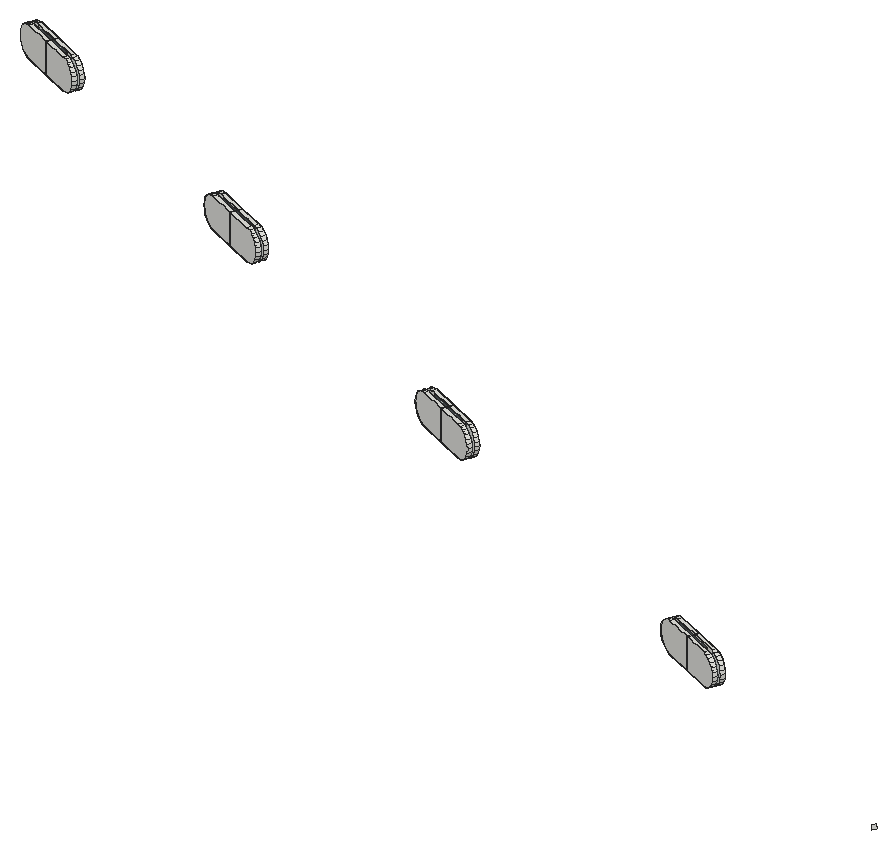
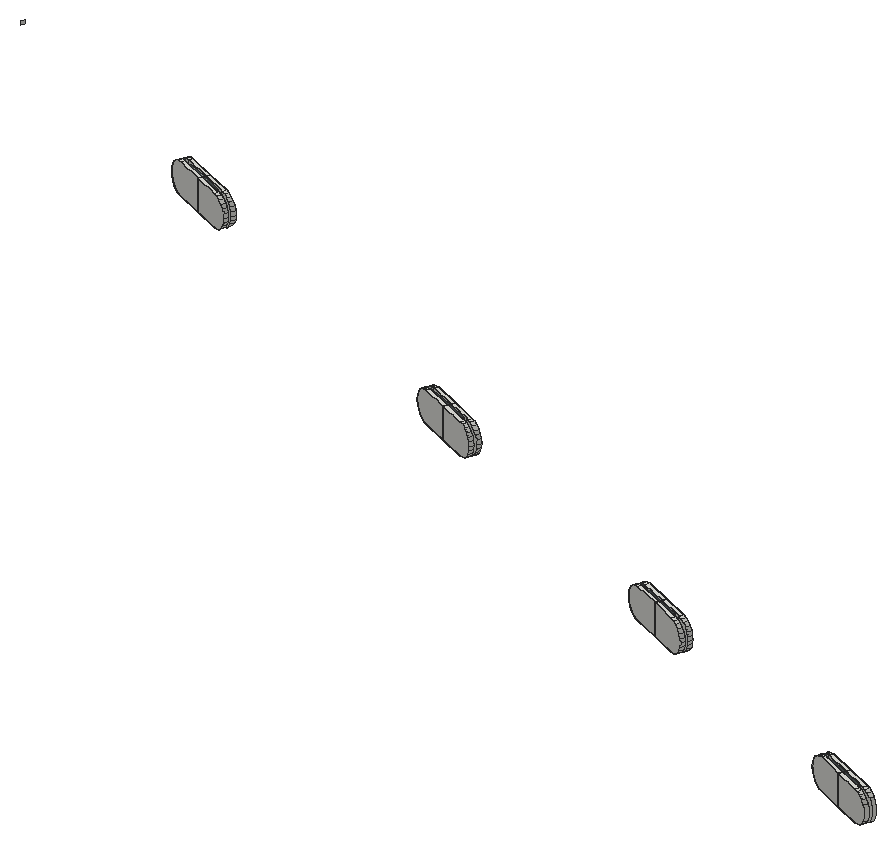
# SketchUp Ruby script. Lengths in inches.
U = 1.inch
M = Sketchup.active_model
def pt(a) = Geom::Point3d.new(a.map { |v| v * U })
def face(e, loops, mat)
  f = e.add_face(loops[0].map { |a| pt(a) })
  loops[1..].each { |l| e.add_face(l.map { |a| pt(a) }).erase! }
  f.material = f.back_material = mat if mat
  f
end
# faces: each face lists its corners as indices into pts; further lists are holes
def faces(e, pts, list, mat = nil) = list.each { |f| face(e, (f[0].is_a?(Array) ? f : [f]).map { |l| l.map { |i| pts[i] } }, mat) }
# xy, xz, yz: faces in a plane at the given z, y or x. An outline is a flat list of corners, or four numbers for a rectangle; further outlines are holes
def ring(l) = l.size == 4 ? [[l[0], l[1]], [l[2], l[1]], [l[2], l[3]], [l[0], l[3]]] : l.each_slice(2).to_a
def flat(e, list, mat, &to3) = list.each { |f| face(e, (f[0].is_a?(Array) ? f : [f]).map { |l| ring(l).map { |u, v| to3.(u, v) } }, mat) }
def xy(e, z, list, mat = nil) = flat(e, list, mat) { |x, y| [x, y, z] }
def xz(e, y, list, mat = nil) = flat(e, list, mat) { |x, z| [x, y, z] }
def yz(e, x, list, mat = nil) = flat(e, list, mat) { |y, z| [x, y, z] }
def lines(e, pts, list) = list.each { |a, b| e.add_line(pt(pts[a]), pt(pts[b])) }
# prism: a flat outline (further loops are holes) pulled along v
def prism(e, loops, v, mat = nil)
  f = face(e, loops, mat); d = Geom::Vector3d.new(v.map { |x| x * U })
  f.pushpull(f.normal.samedirection?(d) ? d.length : -d.length)
end
def box(e, o, s, mat = nil) = prism(e, [[o, [o[0] + s[0], o[1], o[2]], [o[0] + s[0], o[1] + s[1], o[2]], [o[0], o[1] + s[1], o[2]]]], [0, 0, s[2]], mat)
def at(x, y, z, deg = 0) = Geom::Transformation.translation(pt([x, y, z])) * Geom::Transformation.rotation(ORIGIN, Z_AXIS, deg.degrees)
def axes(o, x, y, z) = Geom::Transformation.new([*x, 0, *y, 0, *z, 0, *pt(o).to_a, 1])
def part(name) = M.definitions.add(name)
# library, detail: a bought-in or finely detailed component or shape, given as its bounding box
def library(name, o, s) = part(name).tap { |d| box(d.entities, o, s) }
def detail(e, o, s) = box(e.add_group.entities, o, s)
def put(e, d, t, mat = nil) = e.add_instance(d, t).tap { |i| i.material = mat if mat }
def group(e, t, mat = nil) = e.add_group.tap { |g| g.transformation = t; g.material = mat if mat }.entities
root = M.entities
M.materials.add("Glass_Safety_01").color = [204, 235, 244]
M.materials["Glass_Safety_01"].alpha = 0.1
xy(root,333,[[702.16,595.06,700.36,595.84,700.47,596.09,702.27,595.31],[702.35,595.49,700.55,596.28,700.66,596.53,702.46,595.74],[700.36,595.84,698.55,596.63,698.66,596.88,698.79,596.83,700.47,596.09],[700.55,596.28,698.87,597.01,698.74,597.0625,698.85,597.3125,700.66,596.53],[675.93,606.48,674.12,607.27,674.23,607.52,676.04,606.74],
  [676.12,606.92,674.3125,607.7,674.42,607.95,676.23,607.17],[674.12,607.27,672.32,608.05,672.43,608.31,672.57,608.24,674.23,607.52],[674.3125,607.7,672.65,608.43,672.51,608.49,672.62,608.74,674.42,607.95],[653.36,616.3125,651.55,617.1,651.66,617.35,653.47,616.57],[653.55,616.75,651.74,617.53,651.85,617.78,653.66,617],
  [651.55,617.1,649.75,617.88,649.86,618.14,650.02,618.07,651.66,617.35],[651.74,617.53,650.1,618.25,649.9375,618.32,650.05,618.57,651.85,617.78],[633.71,624.87,631.91,625.65,632.02,625.91,633.82,625.12],[633.9,625.3,632.1,626.09,632.21,626.34,634.01,625.55],[631.91,625.65,630.1,626.44,630.21,626.69,630.38,626.62,632.02,625.91],
  [632.1,626.09,630.46,626.8,630.29,626.875,630.4,627.125,632.21,626.34]])
xy(root,333.08,[[701.91,595.47,700.47,596.09,700.55,596.28,701.99,595.65],[700.47,596.09,699.03,596.72,699.1,596.9,700.55,596.28],[675.68,606.89,674.23,607.52,674.3125,607.7,675.76,607.07],[674.23,607.52,672.79,608.15,672.87,608.33,674.3125,607.7],[653.11,616.72,651.66,617.35,651.74,617.53,653.19,616.9],
  [651.66,617.35,650.22,617.98,650.3,618.16,651.74,617.53],[633.46,625.28,632.02,625.91,632.1,626.09,633.54,625.46],[632.02,625.91,630.57,626.54,630.65,626.72,632.1,626.09]],"Glass_Safety_01")
xy(root,335.05,[[701.91,595.47,701.99,595.65,700.55,596.28,700.47,596.09],[700.47,596.09,700.55,596.28,699.1,596.9,699.03,596.72],[675.68,606.89,675.76,607.07,674.3125,607.7,674.23,607.52],[674.23,607.52,674.3125,607.7,672.87,608.33,672.79,608.15],[653.11,616.72,653.19,616.9,651.74,617.53,651.66,617.35],
  [651.66,617.35,651.74,617.53,650.3,618.16,650.22,617.98],[633.46,625.28,633.54,625.46,632.1,626.09,632.02,625.91],[632.02,625.91,632.1,626.09,630.65,626.72,630.57,626.54]],"Glass_Safety_01")
xy(root,335.125,[[702.16,595.06,702.27,595.31,700.47,596.09,700.36,595.84],[702.35,595.49,702.46,595.74,700.66,596.53,700.55,596.28],[700.36,595.84,700.47,596.09,698.79,596.83,698.66,596.88,698.55,596.63],[700.55,596.28,700.66,596.53,698.85,597.3125,698.74,597.0625,698.87,597.01],[675.93,606.48,676.04,606.74,674.23,607.52,674.12,607.27],
  [676.12,606.92,676.23,607.17,674.42,607.95,674.3125,607.7],[674.12,607.27,674.23,607.52,672.57,608.24,672.43,608.31,672.32,608.05],[674.3125,607.7,674.42,607.95,672.62,608.74,672.51,608.49,672.65,608.43],[653.36,616.3125,653.47,616.57,651.66,617.35,651.55,617.1],[653.55,616.75,653.66,617,651.85,617.78,651.74,617.53],
  [651.55,617.1,651.66,617.35,650.02,618.07,649.86,618.14,649.75,617.88],[651.74,617.53,651.85,617.78,650.05,618.57,649.9375,618.32,650.1,618.25],[633.71,624.87,633.82,625.12,632.02,625.91,631.91,625.65],[633.9,625.3,634.01,625.55,632.21,626.34,632.1,626.09],[631.91,625.65,632.02,625.91,630.38,626.62,630.21,626.69,630.1,626.44],
  [632.1,626.09,632.21,626.34,630.4,627.125,630.29,626.875,630.46,626.8]])
p = [[702.16,595.06,335.125],[700.36,595.84,335.125],[700.36,595.84,333],[702.16,595.06,333],[702.42,594.95,333.04],[702.65,594.84,333.14],
  [702.85,594.76,333.3125],[703.01,594.6875,333.53],[703.11,594.65,333.79],[703.14,594.63,334.0625],[703.11,594.65,334.34],[703.01,594.6875,334.59],
  [702.85,594.76,334.8125],[702.65,594.84,334.98],[702.42,594.95,335.09],[702.53,595.2,333.04],[702.76,595.1,333.14],[702.27,595.31,333],
  [702.27,595.31,335.125],[702.96,595.01,333.3125],[703.12,594.94,333.53],[703.22,594.9,333.79],[703.25,594.88,334.0625],[703.22,594.9,334.34],
  [703.12,594.94,334.59],[702.96,595.01,334.8125],[702.76,595.1,334.98],[702.53,595.2,335.09],[702.35,595.49,333],[702.35,595.49,335.125],
  [702.61,595.38,335.09],[702.84,595.28,334.98],[703.04,595.1875,334.8125],[703.2,595.12,334.59],[703.29,595.08,334.34],[703.33,595.06,334.0625],
  [703.29,595.08,333.79],[703.2,595.12,333.53],[703.04,595.1875,333.3125],[702.84,595.28,333.14],[702.61,595.38,333.04],[700.47,596.09,335.125],
  [700.47,596.09,333],[700.47,596.09,333.08],[701.91,595.47,333.08],[701.91,595.47,335.05],[700.47,596.09,335.05],[700.66,596.53,335.125],
  [702.46,595.74,335.125],[702.72,595.63,335.09],[702.95,595.53,334.98],[703.15,595.44,334.8125],[703.31,595.375,334.59],[703.4,595.33,334.34],
  [703.4375,595.32,334.0625],[703.4,595.33,333.79],[703.31,595.375,333.53],[703.15,595.44,333.3125],[702.95,595.53,333.14],[702.72,595.63,333.04],
  [702.46,595.74,333],[700.66,596.53,333],[700.55,596.28,333],[700.55,596.28,335.125],[700.55,596.28,335.05],[701.99,595.65,335.05],
  [701.99,595.65,333.08],[700.55,596.28,333.08],[698.55,596.63,335.125],[698.3,596.74,335.09],[698.07,596.84,334.98],[697.87,596.93,334.8125],
  [697.71,597,334.59],[697.61,597.04,334.34],[697.58,597.05,334.0625],[697.61,597.04,333.79],[697.71,597,333.53],[697.87,596.93,333.3125],
  [698.07,596.84,333.14],[698.3,596.74,333.04],[698.55,596.63,333],[698.79,596.83,333],[698.79,596.83,335.125],[699.03,596.72,335.05],
  [699.03,596.72,333.08],[698.87,597.01,335.125],[698.87,597.01,333],[699.1,596.9,333.08],[699.1,596.9,335.05],[698.85,597.3125,335.125],
  [698.85,597.3125,333],[698.6,597.42,333.04],[698.37,597.53,333.14],[698.16,597.61,333.3125],[698.01,597.68,333.53],[697.91,597.72,333.79],
  [697.88,597.74,334.0625],[697.91,597.72,334.34],[698.01,597.68,334.59],[698.16,597.61,334.8125],[698.37,597.53,334.98],[698.6,597.42,335.09],
  [698.41,596.99,333.04],[698.66,596.88,333],[698.18,597.09,333.14],[698.66,596.88,335.125],[697.98,597.18,333.3125],[697.82,597.25,333.53],
  [697.72,597.29,333.79],[697.69,597.31,334.0625],[697.72,597.29,334.34],[697.82,597.25,334.59],[697.98,597.18,334.8125],[698.18,597.09,334.98],
  [698.41,596.99,335.09],[698.74,597.0625,333],[698.74,597.0625,335.125],[698.49,597.17,335.09],[698.26,597.27,334.98],[698.05,597.36,334.8125],
  [697.9,597.43,334.59],[697.8,597.47,334.34],[697.77,597.49,334.0625],[697.8,597.47,333.79],[697.9,597.43,333.53],[698.05,597.36,333.3125],
  [698.26,597.27,333.14],[698.49,597.17,333.04],[675.93,606.48,335.125],[674.12,607.27,335.125],[674.12,607.27,333],[675.93,606.48,333],
  [676.18,606.37,333.04],[676.41,606.27,333.14],[676.62,606.18,333.3125],[676.77,606.12,333.53],[676.87,606.07,333.79],[676.9,606.06,334.0625],
  [676.87,606.07,334.34],[676.77,606.12,334.59],[676.62,606.18,334.8125],[676.41,606.27,334.98],[676.18,606.37,335.09],[676.04,606.74,335.125],
  [676.04,606.74,333],[676.29,606.625,333.04],[676.52,606.52,333.14],[676.73,606.44,333.3125],[676.88,606.37,333.53],[676.98,606.33,333.79],
  [677.01,606.3125,334.0625],[676.98,606.33,334.34],[676.88,606.37,334.59],[676.73,606.44,334.8125],[676.52,606.52,334.98],[676.29,606.625,335.09],
  [676.12,606.92,333],[676.12,606.92,335.125],[676.37,606.81,335.09],[676.6,606.7,334.98],[676.81,606.62,334.8125],[676.96,606.55,334.59],
  [677.06,606.51,334.34],[677.09,606.49,334.0625],[677.06,606.51,333.79],[676.96,606.55,333.53],[676.81,606.62,333.3125],[676.6,606.7,333.14],
  [676.37,606.81,333.04],[674.23,607.52,335.125],[674.23,607.52,333],[674.23,607.52,333.08],[675.68,606.89,333.08],[675.68,606.89,335.05],
  [674.23,607.52,335.05],[674.42,607.95,335.125],[676.23,607.17,335.125],[676.48,607.06,335.09],[676.71,606.96,334.98],[676.92,606.87,334.8125],
  [677.07,606.8,334.59],[677.17,606.76,334.34],[677.2,606.74,334.0625],[677.17,606.76,333.79],[677.07,606.8,333.53],[676.92,606.87,333.3125],
  [676.71,606.96,333.14],[676.48,607.06,333.04],[676.23,607.17,333],[674.42,607.95,333],[674.3125,607.7,333],[674.3125,607.7,335.125],
  [674.3125,607.7,335.05],[675.76,607.07,335.05],[675.76,607.07,333.08],[674.3125,607.7,333.08],[672.32,608.05,335.125],[672.07,608.16,335.09],
  [671.83,608.27,334.98],[671.63,608.36,334.8125],[671.47,608.42,334.59],[671.375,608.46,334.34],[671.34,608.48,334.0625],[671.375,608.46,333.79],
  [671.47,608.42,333.53],[671.63,608.36,333.3125],[671.83,608.27,333.14],[672.07,608.16,333.04],[672.32,608.05,333],[672.57,608.24,333],
  [672.57,608.24,335.125],[672.79,608.15,335.05],[672.79,608.15,333.08],[672.65,608.43,335.125],[672.65,608.43,333],[672.87,608.33,333.08],
  [672.87,608.33,335.05],[672.62,608.74,335.125],[672.62,608.74,333],[672.36,608.85,333.04],[672.13,608.95,333.14],[671.93,609.04,333.3125],
  [671.77,609.11,333.53],[671.68,609.15,333.79],[671.64,609.17,334.0625],[671.68,609.15,334.34],[671.77,609.11,334.59],[671.93,609.04,334.8125],
  [672.13,608.95,334.98],[672.36,608.85,335.09],[672.18,608.42,333.04],[672.43,608.31,333],[672.43,608.31,335.125],[671.94,608.52,333.14],
  [671.74,608.61,333.3125],[671.58,608.68,333.53],[671.49,608.72,333.79],[671.45,608.73,334.0625],[671.49,608.72,334.34],[671.58,608.68,334.59],
  [671.74,608.61,334.8125],[671.94,608.52,334.98],[672.18,608.42,335.09],[672.51,608.49,333],[672.51,608.49,335.125],[672.25,608.6,335.09],
  [672.02,608.7,334.98],[671.82,608.79,334.8125],[671.66,608.86,334.59],[671.57,608.9,334.34],[671.53,608.91,334.0625],[671.57,608.9,333.79],
  [671.66,608.86,333.53],[671.82,608.79,333.3125],[672.02,608.7,333.14],[672.25,608.6,333.04],[653.36,616.3125,335.125],[651.55,617.1,335.125],
  [651.55,617.1,333],[653.36,616.3125,333],[653.61,616.2,333.04],[653.84,616.1,333.14],[654.05,616.01,333.3125],[654.2,615.95,333.53],
  [654.3,615.9,333.79],[654.33,615.89,334.0625],[654.3,615.9,334.34],[654.2,615.95,334.59],[654.05,616.01,334.8125],[653.84,616.1,334.98],
  [653.61,616.2,335.09],[653.47,616.57,335.125],[653.47,616.57,333],[653.72,616.46,333.04],[653.96,616.35,333.14],[654.16,616.27,333.3125],
  [654.3125,616.2,333.53],[654.41,616.16,333.79],[654.44,616.14,334.0625],[654.41,616.16,334.34],[654.3125,616.2,334.59],[654.16,616.27,334.8125],
  [653.96,616.35,334.98],[653.72,616.46,335.09],[653.55,616.75,333],[653.55,616.75,335.125],[653.8,616.64,335.09],[654.03,616.53,334.98],
  [654.24,616.45,334.8125],[654.39,616.38,334.59],[654.49,616.34,334.34],[654.52,616.32,334.0625],[654.49,616.34,333.79],[654.39,616.38,333.53],
  [654.24,616.45,333.3125],[654.03,616.53,333.14],[653.8,616.64,333.04],[653.91,616.89,333.04],[654.14,616.79,333.14],[651.66,617.35,335.125],
  [651.66,617.35,333],[651.66,617.35,333.08],[653.11,616.72,333.08],[653.11,616.72,335.05],[651.66,617.35,335.05],[651.85,617.78,335.125],
  [653.66,617,335.125],[653.91,616.89,335.09],[654.14,616.79,334.98],[654.35,616.7,334.8125],[654.5,616.63,334.59],[654.6,616.59,334.34],
  [654.63,616.57,334.0625],[654.6,616.59,333.79],[654.5,616.63,333.53],[654.35,616.7,333.3125],[653.66,617,333],[651.85,617.78,333],
  [651.74,617.53,333],[651.74,617.53,335.125],[651.74,617.53,335.05],[653.19,616.9,335.05],[653.19,616.9,333.08],[651.74,617.53,333.08],
  [649.75,617.88,335.125],[649.5,617.99,335.09],[649.26,618.1,334.98],[649.06,618.18,334.8125],[648.9,618.25,334.59],[648.81,618.29,334.34],
  [648.77,618.31,334.0625],[648.81,618.29,333.79],[648.9,618.25,333.53],[649.06,618.18,333.3125],[649.26,618.1,333.14],[649.5,617.99,333.04],
  [649.75,617.88,333],[650.02,618.07,333],[650.02,618.07,335.125],[650.22,617.98,335.05],[650.22,617.98,333.08],[650.1,618.25,335.125],
  [650.1,618.25,333],[650.3,618.16,333.08],[650.3,618.16,335.05],[650.05,618.57,335.125],[650.05,618.57,333],[649.79,618.68,333.04],
  [649.56,618.78,333.14],[649.36,618.87,333.3125],[649.2,618.9375,333.53],[649.11,618.98,333.79],[649.07,618.99,334.0625],[649.11,618.98,334.34],
  [649.2,618.9375,334.59],[649.36,618.87,334.8125],[649.56,618.78,334.98],[649.79,618.68,335.09],[649.61,618.25,333.04],[649.86,618.14,333],
  [649.37,618.35,333.14],[649.86,618.14,335.125],[649.17,618.4375,333.3125],[649.01,618.5,333.53],[648.92,618.55,333.79],[648.88,618.5625,334.0625],
  [648.92,618.55,334.34],[649.01,618.5,334.59],[649.17,618.4375,334.8125],[649.37,618.35,334.98],[649.61,618.25,335.09],[649.9375,618.32,333],
  [649.9375,618.32,335.125],[649.68,618.43,335.09],[649.45,618.53,334.98],[649.25,618.62,334.8125],[649.09,618.69,334.59],[649,618.73,334.34],
  [648.96,618.74,334.0625],[649,618.73,333.79],[649.09,618.69,333.53],[649.25,618.62,333.3125],[649.45,618.53,333.14],[649.68,618.43,333.04],
  [633.71,624.87,335.125],[631.91,625.65,335.125],[631.91,625.65,333],[633.71,624.87,333],[633.96,624.76,333.04],[634.2,624.66,333.14],
  [634.4,624.57,333.3125],[634.56,624.5,333.53],[634.65,624.46,333.79],[634.6875,624.44,334.0625],[634.65,624.46,334.34],[634.56,624.5,334.59],
  [634.4,624.57,334.8125],[634.2,624.66,334.98],[633.96,624.76,335.09],[633.82,625.12,335.125],[633.82,625.12,333],[634.07,625.01,333.04],
  [634.31,624.91,333.14],[634.51,624.82,333.3125],[634.67,624.75,333.53],[634.76,624.71,333.79],[634.8,624.7,334.0625],[634.76,624.71,334.34],
  [634.67,624.75,334.59],[634.51,624.82,334.8125],[634.31,624.91,334.98],[634.07,625.01,335.09],[633.9,625.3,333],[633.9,625.3,335.125],
  [634.15,625.19,335.09],[634.39,625.09,334.98],[634.59,625,334.8125],[634.75,624.93,334.59],[634.84,624.89,334.34],[634.875,624.88,334.0625],
  [634.84,624.89,333.79],[634.75,624.93,333.53],[634.59,625,333.3125],[634.39,625.09,333.14],[634.15,625.19,333.04],[632.02,625.91,335.125],
  [632.02,625.91,333],[632.02,625.91,333.08],[633.46,625.28,333.08],[633.46,625.28,335.05],[632.02,625.91,335.05],[632.21,626.34,335.125],
  [634.01,625.55,335.125],[634.26,625.44,335.09],[634.5,625.34,334.98],[634.7,625.25,334.8125],[634.86,625.1875,334.59],[634.95,625.14,334.34],
  [634.99,625.13,334.0625],[634.95,625.14,333.79],[634.86,625.1875,333.53],[634.7,625.25,333.3125],[634.5,625.34,333.14],[634.26,625.44,333.04],
  [634.01,625.55,333],[632.21,626.34,333],[632.1,626.09,333],[632.1,626.09,335.125],[632.1,626.09,335.05],[633.54,625.46,335.05],
  [633.54,625.46,333.08],[632.1,626.09,333.08],[630.1,626.44,335.125],[629.85,626.55,335.09],[629.62,626.65,334.98],[629.41,626.74,334.8125],
  [629.26,626.81,334.59],[629.16,626.85,334.34],[629.13,626.87,334.0625],[629.16,626.85,333.79],[629.26,626.81,333.53],[629.41,626.74,333.3125],
  [629.62,626.65,333.14],[629.85,626.55,333.04],[630.1,626.44,333],[630.38,626.62,333],[630.38,626.62,335.125],[630.57,626.54,335.05],
  [630.57,626.54,333.08],[630.46,626.8,335.125],[630.46,626.8,333],[630.65,626.72,333.08],[630.65,626.72,335.05],[630.4,627.125,335.125],
  [630.4,627.125,333],[630.15,627.24,333.04],[629.91,627.34,333.14],[629.71,627.43,333.3125],[629.56,627.49,333.53],[629.46,627.54,333.79],
  [629.43,627.55,334.0625],[629.46,627.54,334.34],[629.56,627.49,334.59],[629.71,627.43,334.8125],[629.91,627.34,334.98],[630.15,627.24,335.09],
  [629.96,626.8,333.04],[630.21,626.69,333],[630.21,626.69,335.125],[629.73,626.91,333.14],[629.52,626.99,333.3125],[629.37,627.0625,333.53],
  [629.27,627.1,333.79],[629.24,627.12,334.0625],[629.27,627.1,334.34],[629.37,627.0625,334.59],[629.52,626.99,334.8125],[629.73,626.91,334.98],
  [629.96,626.8,335.09],[630.29,626.875,333],[630.29,626.875,335.125],[630.04,626.98,335.09],[629.8,627.09,334.98],[629.6,627.17,334.8125],
  [629.45,627.24,334.59],[629.35,627.28,334.34],[629.32,627.3,334.0625],[629.35,627.28,333.79],[629.45,627.24,333.53],[629.6,627.17,333.3125],
  [629.8,627.09,333.14],[630.04,626.98,333.04],[720.21,587.5,334.0625],[720.24,587.48,333.79],[720.13,587.23,333.79],[720.1,587.25,334.0625]]
faces(root,p,[[0,1,2,3,4,5,6,7,8,9,10,11,12,13,14],[15,16,5,4],[17,15,4,3],[41,18,17,42,43,44,45,46],[47,48,49,50,51,52,53,54,55,56,57,58,59,60,61],[39,40,59,58],[40,28,60,59],[62,28,29,63,64,65,66,67],
  [1,68,69,70,71,72,73,74,75,76,77,78,79,80,2],[42,43,46,41,1,2],[42,81,82,41,46,83,84,43],[63,85,86,62,67,87,88,64],[67,62,61,47,63,64],[89,47,61,90,91,92,93,94,95,96,97,98,99,100,101],[102,103,80,79],[104,102,79,78],
  [105,82,81,103,102,104,106,107,108,109,110,111,112,113,114],[115,86,85,116,117,118,119,120,121,122,123,124,125,126,127],[115,127,91,90],[127,126,92,91],[128,129,130,131,132,133,134,135,136,137,138,139,140,141,142],[145,146,133,132],[144,145,132,131],[169,143,144,170,171,172,173,174],
  [175,176,177,178,179,180,181,182,183,184,185,186,187,188,189],[167,168,187,186],[168,156,188,187],[190,156,157,191,192,193,194,195],[129,196,197,198,199,200,201,202,203,204,205,206,207,208,130],[170,171,174,169,129,130],[170,209,210,169,174,211,212,171],[191,213,214,190,195,215,216,192],
  [195,190,189,175,191,192],[217,175,189,218,219,220,221,222,223,224,225,226,227,228,229],[230,231,208,207],[232,210,209,231,230,233,234,235,236,237,238,239,240,241,242],[233,230,207,206],[243,214,213,244,245,246,247,248,249,250,251,252,253,254,255],[243,255,219,218],[255,254,220,219],
  [256,257,258,259,260,261,262,263,264,265,266,267,268,269,270],[273,274,261,260],[272,273,260,259],[295,296,297,298],[299,271,272,300,301,302,303,304],[305,306,307,308,309,310,311,312,313,314,315,298,297,316,317],[296,284,316,297],[318,284,285,319,320,321,322,323],
  [257,324,325,326,327,328,329,330,331,332,333,334,335,336,258],[300,301,304,299,257,258],[300,337,338,299,304,339,340,301],[319,341,342,318,323,343,344,320],[323,318,317,305,319,320],[345,305,317,346,347,348,349,350,351,352,353,354,355,356,357],[358,359,336,335],[360,358,335,334],
  [361,338,337,359,358,360,362,363,364,365,366,367,368,369,370],[371,342,341,372,373,374,375,376,377,378,379,380,381,382,383],[371,383,347,346],[383,382,348,347],[384,385,386,387,388,389,390,391,392,393,394,395,396,397,398],[401,402,389,388],[400,401,388,387],[425,399,400,426,427,428,429,430],
  [431,432,433,434,435,436,437,438,439,440,441,442,443,444,445],[423,424,443,442],[424,412,444,443],[446,412,413,447,448,449,450,451],[385,452,453,454,455,456,457,458,459,460,461,462,463,464,386],[426,427,430,425,385,386],[426,465,466,425,430,467,468,427],[447,469,470,446,451,471,472,448],
  [451,446,445,431,447,448],[473,431,445,474,475,476,477,478,479,480,481,482,483,484,485],[486,487,464,463],[488,466,465,487,486,489,490,491,492,493,494,495,496,497,498],[489,486,463,462],[499,470,469,500,501,502,503,504,505,506,507,508,509,510,511],[499,511,475,474],[511,510,476,475],
  [16,19,6,5],[38,39,58,57],[106,104,78,77],[126,125,93,92],[146,147,134,133],[166,167,186,185],[234,233,206,205],[254,253,221,220],
  [274,275,262,261],[294,295,298,315],[362,360,334,333],[382,381,349,348],[402,403,390,389],[422,423,442,441],[510,509,477,476],[19,20,7,6],
  [37,38,57,56],[107,106,77,76],[125,124,94,93],[147,148,135,134],[165,166,185,184],[235,234,205,204],[253,252,222,221],[275,276,263,262],
  [293,294,315,314],[363,362,333,332],[381,380,350,349],[403,404,391,390],[421,422,441,440],[509,508,478,477],[20,21,8,7],[36,37,56,55],
  [108,107,76,75],[124,123,95,94],[148,149,136,135],[164,165,184,183],[236,235,204,203],[252,251,223,222],[276,277,264,263],[292,293,314,313],
  [364,363,332,331],[380,379,351,350],[404,405,392,391],[420,421,440,439],[512,513,514,515],[21,22,9,8],[35,36,55,54],[109,108,75,74],
  [123,122,96,95],[149,150,137,136],[163,164,183,182],[237,236,203,202],[251,250,224,223],[277,278,265,264],[291,292,313,312],[365,364,331,330],
  [379,378,352,351],[405,406,393,392],[419,420,439,438],[22,23,10,9],[34,35,54,53],[110,109,74,73],[122,121,97,96],[150,151,138,137],
  [162,163,182,181],[238,237,202,201],[250,249,225,224],[278,279,266,265],[290,291,312,311],[366,365,330,329],[378,377,353,352],[406,407,394,393],
  [418,419,438,437],[23,24,11,10],[33,34,53,52],[111,110,73,72],[121,120,98,97],[151,152,139,138],[161,162,181,180],[239,238,201,200],
  [249,248,226,225],[279,280,267,266],[289,290,311,310],[367,366,329,328],[377,376,354,353],[407,408,395,394],[417,418,437,436],[24,25,12,11],
  [32,33,52,51],[112,111,72,71],[120,119,99,98],[152,153,140,139],[160,161,180,179],[240,239,200,199],[248,247,227,226],[280,281,268,267],
  [288,289,310,309],[368,367,328,327],[376,375,355,354],[408,409,396,395],[416,417,436,435],[504,503,483,482],[25,26,13,12],[31,32,51,50],
  [113,112,71,70],[119,118,100,99],[153,154,141,140],[159,160,179,178],[241,240,199,198],[247,246,228,227],[281,282,269,268],[287,288,309,308],
  [369,368,327,326],[375,374,356,355],[409,410,397,396],[415,416,435,434],[497,496,455,454],[503,502,484,483],[26,27,14,13],[30,31,50,49],
  [114,113,70,69],[118,117,101,100],[154,155,142,141],[158,159,178,177],[242,241,198,197],[246,245,229,228],[282,283,270,269],[286,287,308,307],
  [370,369,326,325],[374,373,357,356],[410,411,398,397],[414,415,434,433],[498,497,454,453],[502,501,485,484],[27,18,0,14],[29,30,49,48],
  [105,114,69,68],[117,116,89,101],[155,143,128,142],[157,158,177,176],[232,242,197,196],[245,244,217,229],[283,271,256,270],[285,286,307,306],
  [361,370,325,324],[373,372,345,357],[411,399,384,398],[413,414,433,432],[488,498,453,452],[501,500,473,485]])
faces(root,p,[[18,17,15,16,19,20,21,22,23,24,25,26,27],[28,29,30,31,32,33,34,35,36,37,38,39,40],[143,144,145,146,147,148,149,150,151,152,153,154,155],[156,157,158,159,160,161,162,163,164,165,166,167,168],[271,272,273,274,275,276,277,278,279,280,281,282,283],[284,285,286,287,288,289,290,291,292,293,294,295,296],[399,400,401,402,403,404,405,406,407,408,409,410,411],[412,413,414,415,416,417,418,419,420,421,422,423,424],
  [44,43,46,45],[66,65,45,44],[67,66,65,64],[43,84,83,46],[43,67,64,46],[87,67,64,88],[84,83,88,87],[172,171,174,173],
  [194,193,173,172],[195,194,193,192],[171,212,211,174],[171,195,192,174],[215,195,192,216],[212,211,216,215],[302,301,304,303],[303,302,322,321],
  [323,322,321,320],[301,340,339,304],[320,304,301,323],[343,323,320,344],[340,339,344,343],[428,427,430,429],[429,428,450,449],[451,450,449,448],
  [427,468,467,430],[448,430,427,451],[471,451,448,472],[468,467,472,471]],"Glass_Safety_01")
